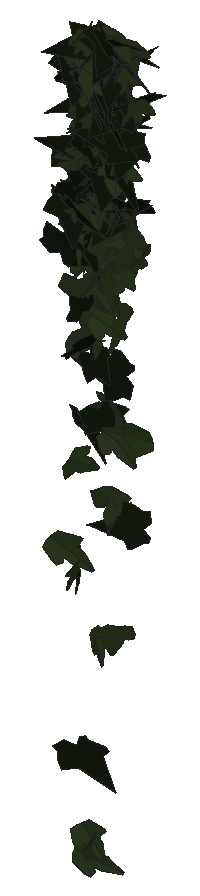
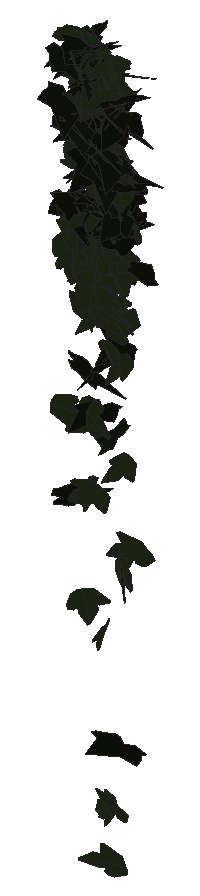
# SketchUp Ruby script. Lengths in inches.
U = 1.inch
M = Sketchup.active_model
def pt(a) = Geom::Point3d.new(a.map { |v| v * U })
def face(e, loops, mat)
  f = e.add_face(loops[0].map { |a| pt(a) })
  loops[1..].each { |l| e.add_face(l.map { |a| pt(a) }).erase! }
  f.material = f.back_material = mat if mat
  f
end
# faces: each face lists its corners as indices into pts; further lists are holes
def faces(e, pts, list, mat = nil) = list.each { |f| face(e, (f[0].is_a?(Array) ? f : [f]).map { |l| l.map { |i| pts[i] } }, mat) }
# xy, xz, yz: faces in a plane at the given z, y or x. An outline is a flat list of corners, or four numbers for a rectangle; further outlines are holes
def ring(l) = l.size == 4 ? [[l[0], l[1]], [l[2], l[1]], [l[2], l[3]], [l[0], l[3]]] : l.each_slice(2).to_a
def flat(e, list, mat, &to3) = list.each { |f| face(e, (f[0].is_a?(Array) ? f : [f]).map { |l| ring(l).map { |u, v| to3.(u, v) } }, mat) }
def xy(e, z, list, mat = nil) = flat(e, list, mat) { |x, y| [x, y, z] }
def xz(e, y, list, mat = nil) = flat(e, list, mat) { |x, z| [x, y, z] }
def yz(e, x, list, mat = nil) = flat(e, list, mat) { |y, z| [x, y, z] }
def lines(e, pts, list) = list.each { |a, b| e.add_line(pt(pts[a]), pt(pts[b])) }
# prism: a flat outline (further loops are holes) pulled along v
def prism(e, loops, v, mat = nil)
  f = face(e, loops, mat); d = Geom::Vector3d.new(v.map { |x| x * U })
  f.pushpull(f.normal.samedirection?(d) ? d.length : -d.length)
end
def box(e, o, s, mat = nil) = prism(e, [[o, [o[0] + s[0], o[1], o[2]], [o[0] + s[0], o[1] + s[1], o[2]], [o[0], o[1] + s[1], o[2]]]], [0, 0, s[2]], mat)
def at(x, y, z, deg = 0) = Geom::Transformation.translation(pt([x, y, z])) * Geom::Transformation.rotation(ORIGIN, Z_AXIS, deg.degrees)
def axes(o, x, y, z) = Geom::Transformation.new([*x, 0, *y, 0, *z, 0, *pt(o).to_a, 1])
def part(name) = M.definitions.add(name)
# library, detail: a bought-in or finely detailed component or shape, given as its bounding box
def library(name, o, s) = part(name).tap { |d| box(d.entities, o, s) }
def detail(e, o, s) = box(e.add_group.entities, o, s)
def put(e, d, t, mat = nil) = e.add_instance(d, t).tap { |i| i.material = mat if mat }
def group(e, t, mat = nil) = e.add_group.tap { |g| g.transformation = t; g.material = mat if mat }.entities
root = M.entities
M.materials.add("1026 AP 7946 SUNNY SIDE UP").color = [254, 231, 186]
M.materials.add("efeu1").color = [18, 25, 13]
M.materials.add("efeu2").color = [43, 57, 29]
c1 = part("ivyleaf_10")
p = [[0,0.5,-0.03],[-0.0625,2.02,-0.43],[-0.19,2.01,-0.46],[-0.54,1.05,-0.29],[-0.52,0.625,-0.18],[-0.83,0.76,-0.28],
  [-1.16,0.64,-0.33],[-1.15,0.33,-0.24],[-0.77,-0.39,0.02],[-0.3,-0.51,0.16],[0.04,-0.48,0.23],[-0.02,2.01,-0.4375],
  [-0.06,2.01,-0.43],[0.04,-0.49,0.23],[0.67,-0.49,0.14],[1.38,0.36,-0.2],[1.375,0.51,-0.24],[0.81,0.65,-0.19],
  [0.62,0.59,-0.15],[0.6,1.09,-0.28],[0.5,1.23,-0.31]]
faces(c1.entities,p,[[0,1,2,3,4,5,6,7,8,9,10],[11,12,0,13,14,15,16,17,18,19,20]],"efeu2")
c2 = part("ivyleaf_9")
p = [[1.54,2.16,1.25],[1.36,2.04,1.19],[-0.21,0.99,0.68],[-0.71,1.11,0.82],[-0.85,0.86,0.67],[-0.8,0.17,0.21],
  [-0.9,-0.01,0.1],[-0.67,-0.16,-0.02],[-0.08,-0.08,-0.05],[-0.03,-0.6,-0.4],[0.65,-0.88,-0.66],[0.83,-0.6,-0.49],
  [1.29,-0.42,-0.43],[1.8125,-0.07,-0.26],[1.21,0.44,0.15]]
faces(c2.entities,p,[[0,1,2,3,4,5,6,7,8,9,10,11,12,13,14]],"efeu1")
put(root,c1,axes([111.84,212.82,261.67],[0.05347,0.09968,0.2103],[-0.0247,0.20639,-0.1002],[-0.35554,0.00065,0.03859]),"1026 AP 7946 SUNNY SIDE UP")
put(root,c1,axes([111.73,212.95,262.55],[-0.1793,-0.09054,0.18329],[0.19266,0.13077,0.14979],[-0.24874,0.16655,-0.0161]),"1026 AP 7946 SUNNY SIDE UP")
put(root,c1,axes([111.68,212.8,264.51],[0.19312,-0.08424,0.20605],[0.27212,-0.10156,-0.15378],[0.20706,0.21205,0.00993]),"1026 AP 7946 SUNNY SIDE UP")
put(root,c2,axes([111.71,212.66,263.4],[-0.15918,0.06277,0.23387],[0.27221,-0.14715,0.12078],[0.25034,0.19992,0.01739]),"1026 AP 7946 SUNNY SIDE UP")
put(root,c1,axes([111.9375,212.88,265.25],[-0.22565,-0.19814,0.03871],[0.0203,-0.05639,-0.24844],[0.31679,-0.13752,0.04349]),"1026 AP 7946 SUNNY SIDE UP")
put(root,c1,axes([111.9,212.98,263.45],[0.25063,0.14947,-0.07542],[-0.0695,-0.06092,-0.22504],[-0.25292,0.16486,-0.01289]),"1026 AP 7946 SUNNY SIDE UP")
put(root,c2,axes([111.92,212.84,264.66],[0.15143,0.18297,0.13568],[0.05681,0.1277,-0.21091],[-0.34894,0.1002,0.02454]),"1026 AP 7946 SUNNY SIDE UP")
put(root,c2,axes([111.79,212.9,265.29],[-0.05234,-0.20603,-0.13394],[0.07477,0.12201,-0.21294],[0.37471,-0.05312,0.02378]),"1026 AP 7946 SUNNY SIDE UP")
put(root,c2,axes([111.87,212.83,266.68],[0.35119,0.10595,-0.05184],[-0.07077,-0.02394,-0.2548],[-0.17076,0.22783,-0.00102]),"1026 AP 7946 SUNNY SIDE UP")
put(root,c2,axes([111.77,212.91,264.72],[0.35156,-0.09277,-0.03747],[-0.06444,-0.00557,-0.2485],[0.14248,0.22637,-0.01992]),"1026 AP 7946 SUNNY SIDE UP")
put(root,c2,axes([111.86,212.72,264.35],[-0.08105,-0.23623,-0.0209],[0.00422,0.01881,-0.24897],[0.37261,-0.05159,-0.00173]),"1026 AP 7946 SUNNY SIDE UP")
put(root,c2,axes([112.11,212.61,257.58],[0.02333,-0.01712,-0.2645],[-0.35789,0.11888,-0.02103],[0.1884,0.22794,-0.0072]),"1026 AP 7946 SUNNY SIDE UP")
put(root,c2,axes([112.29,212.79,265.43],[-0.25261,0.05653,0.19369],[-0.29315,0.03089,-0.1738],[-0.0952,-0.24512,0.02123]),"1026 AP 7946 SUNNY SIDE UP")
put(root,c1,axes([112.07,212.89,263.88],[-0.3228,-0.10284,0.05543],[-0.06409,-0.03974,-0.23614],[0.17134,-0.20862,0.01609]),"1026 AP 7946 SUNNY SIDE UP")
put(root,c2,axes([112.02,212.92,265.84],[0.11278,0.23174,0.05889],[0.00151,0.05804,-0.24904],[-0.37482,0.06996,0.01672]),"1026 AP 7946 SUNNY SIDE UP")
put(root,c2,axes([111.94,212.91,266.96],[-0.17224,-0.22985,0.01436],[0.00515,-0.01844,-0.26217],[0.36217,-0.10905,0.01056]),"1026 AP 7946 SUNNY SIDE UP")
put(root,c1,axes([112.02,212.9,267.59],[0.04144,-0.25472,0.00311],[-0.00158,-0.00459,-0.26383],[0.40057,0.02633,-0.00136]),"1026 AP 7946 SUNNY SIDE UP")
put(root,c1,axes([111.7,212.58,257.88],[0.19267,0.0524,0.22442],[0.31832,0.07972,-0.13678],[-0.14992,0.23661,-0.00201]),"1026 AP 7946 SUNNY SIDE UP")
put(root,c1,axes([112.01,212.73,257.52],[0.07038,-0.22464,0.05688],[0.00922,-0.05642,-0.23624],[0.36411,0.04485,-0.00501]),"1026 AP 7946 SUNNY SIDE UP")
put(root,c1,axes([111.91,212.93,262.66],[0.29752,-0.11125,0.0746],[0.09033,-0.04626,-0.22615],[0.18878,0.19748,-0.00937]),"1026 AP 7946 SUNNY SIDE UP")
put(root,c2,axes([111.83,212.82,266.94],[0.14158,-0.2361,-0.04521],[-0.01502,0.04187,-0.26],[0.37693,0.09035,0.00662]),"1026 AP 7946 SUNNY SIDE UP")
put(root,c1,axes([112.02,212.89,263.32],[0.21001,-0.18855,0.01303],[-0.01077,-0.02161,-0.23744],[0.29707,0.13251,-0.01782]),"1026 AP 7946 SUNNY SIDE UP")
put(root,c2,axes([112.19,212.8,264.88],[-0.24343,0.18812,-0.066],[0.04972,-0.05823,-0.25102],[-0.30905,-0.15754,0.0116]),"1026 AP 7946 SUNNY SIDE UP")
put(root,c2,axes([111.75,212.65,264.375],[0.24648,-0.13163,0.16154],[0.16019,-0.12223,-0.21034],[0.28027,0.18562,-0.02184]),"1026 AP 7946 SUNNY SIDE UP")
put(root,c2,axes([112.28,212.73,266.5],[-0.33099,0.13407,-0.02675],[-0.02296,-0.07085,-0.24801],[-0.21372,-0.20001,0.06808]),"1026 AP 7946 SUNNY SIDE UP")
put(root,c1,axes([112.18,213.07,262.85],[0.0741,0.09275,-0.20945],[-0.21602,-0.15253,-0.10511],[-0.2781,0.1432,0.02584]),"1026 AP 7946 SUNNY SIDE UP")
put(root,c2,axes([112.3,212.9,267.4],[-0.34884,-0.00818,0.12883],[-0.16792,-0.12088,-0.20395],[0.10326,-0.22418,0.10357]),"1026 AP 7946 SUNNY SIDE UP")
put(root,c1,axes([112,212.62,259.56],[-0.08616,-0.13069,-0.21033],[0.16378,0.17548,-0.14401],[0.3431,-0.11658,0.01593]),"1026 AP 7946 SUNNY SIDE UP")
put(root,c1,axes([111.88,212.92,262.28],[0.18885,-0.09889,-0.17595],[0.23298,-0.08589,0.15859],[-0.20382,-0.18981,0.01826]),"1026 AP 7946 SUNNY SIDE UP")
put(root,c1,axes([112.24,212.85,261.88],[0.19717,-0.1101,-0.16509],[-0.16993,0.11815,-0.17072],[0.25317,0.16506,0.01398]),"1026 AP 7946 SUNNY SIDE UP")
put(root,c2,axes([111.98,212.89,266.46],[0.38487,-0.02762,-0.05832],[-0.08989,-0.0036,-0.25358],[0.04103,0.25116,-0.00856]),"1026 AP 7946 SUNNY SIDE UP")
put(root,c2,axes([111.92,212.83,264.56],[0.3612,-0.07913,-0.02183],[-0.01329,0.03853,-0.24767],[0.12795,0.22741,0.0359]),"1026 AP 7946 SUNNY SIDE UP")
put(root,c1,axes([112.05,212.71,264.27],[-0.2316,-0.15334,-0.12194],[0.16357,0.06154,-0.21672],[0.25595,-0.17808,0.02817]),"1026 AP 7946 SUNNY SIDE UP")
put(root,c1,axes([111.84,213.08,251.79],[0.069,0.02915,0.24774],[0.34727,0.09518,-0.05289],[-0.15585,0.22498,-0.00816]),"1026 AP 7946 SUNNY SIDE UP")
put(root,c1,axes([112.15,212.85,267.56],[0.19577,0.20167,-0.1036],[-0.1137,-0.07444,-0.24367],[-0.33646,0.1425,0.02206]),"1026 AP 7946 SUNNY SIDE UP")
put(root,c1,axes([112.22,212.73,267.1],[-0.40103,-0.03197,0.03618],[-0.04126,-0.06618,-0.25741],[0.0625,-0.24882,0.06224]),"1026 AP 7946 SUNNY SIDE UP")
put(root,c2,axes([111.89,212.8125,264.27],[0.36563,-0.00697,0.07507],[0.11244,-0.03093,-0.23816],[0.02493,0.24172,-0.02687]),"1026 AP 7946 SUNNY SIDE UP")
put(root,c1,axes([112.21,212.76,265.43],[-0.10215,-0.19356,0.14483],[-0.01668,-0.14432,-0.20898],[0.37681,-0.05886,0.03001]),"1026 AP 7946 SUNNY SIDE UP")
put(root,c1,axes([112.25,212.68,265.1875],[-0.26442,-0.16377,0.08131],[-0.06245,-0.07311,-0.24105],[0.27961,-0.1712,0.02306]),"1026 AP 7946 SUNNY SIDE UP")
put(root,c2,axes([112.37,212.9375,265.89],[-0.30157,0.15779,0.00444],[-0.02153,-0.01128,-0.25529],[-0.24723,-0.19149,0.01681]),"1026 AP 7946 SUNNY SIDE UP")
put(root,c1,axes([112.12,212.94,263.83],[-0.22432,-0.17714,-0.07376],[0.10309,0.03723,-0.2325],[0.28155,-0.15476,0.02636]),"1026 AP 7946 SUNNY SIDE UP")
put(root,c2,axes([112.33,212.42,262.63],[-0.05142,0.15685,0.1972],[-0.0844,0.18307,-0.16368],[-0.37875,-0.06209,0.0097]),"1026 AP 7946 SUNNY SIDE UP")
put(root,c2,axes([112.24,212.85,265.39],[0.07253,0.24011,0.03843],[-0.01233,0.03804,-0.2512],[-0.38155,0.04441,0.01542]),"1026 AP 7946 SUNNY SIDE UP")
put(root,c2,axes([111.96,212.93,260.19],[0.13952,-0.22077,0.07776],[0.04322,-0.07165,-0.24554],[0.36496,0.09288,-0.00065]),"1026 AP 7946 SUNNY SIDE UP")
put(root,c2,axes([111.96,212.77,254.01],[-0.06872,-0.10767,-0.23448],[0.28185,0.14808,-0.10705],[0.2768,-0.17751,0.05079]),"1026 AP 7946 SUNNY SIDE UP")
put(root,c1,axes([112.17,212.76,266.47],[-0.07146,-0.24315,-0.04562],[0.10357,0.03011,-0.24747],[0.37417,-0.05477,0.05978]),"1026 AP 7946 SUNNY SIDE UP")
put(root,c2,axes([112.05,212.82,263.71],[0.11511,-0.22771,0.03214],[-0.00401,-0.0349,-0.24625],[0.36166,0.07209,-0.01296]),"1026 AP 7946 SUNNY SIDE UP")
put(root,c2,axes([112.16,212.4375,261.83],[0.13537,0.1643,0.17037],[0.13235,0.14143,-0.19014],[-0.34071,0.12021,-0.00617]),"1026 AP 7946 SUNNY SIDE UP")
put(root,c2,axes([112.35,212.72,265.96],[-0.34043,0.09986,-0.08848],[0.10618,-0.05899,-0.24474],[-0.1785,-0.22554,0.02317]),"1026 AP 7946 SUNNY SIDE UP")
put(root,c1,axes([112.29,212.83,263.73],[-0.1663,-0.18024,0.12665],[-0.02116,-0.13207,-0.21043],[0.34332,-0.09545,0.04838]),"1026 AP 7946 SUNNY SIDE UP")
put(root,c2,axes([112.24,212.77,265.54],[-0.1233,-0.02052,0.25238],[-0.0935,-0.24804,-0.04245],[0.37527,-0.06854,0.07235]),"1026 AP 7946 SUNNY SIDE UP")
put(root,c2,axes([112.08,212.48,264.96],[0.0296,0.07848,-0.27103],[0.03559,0.26281,0.08383],[0.4309,-0.02709,0.01169]),"1026 AP 7946 SUNNY SIDE UP")
put(root,c1,axes([112.32,212.93,266.9],[-0.27535,-0.17364,0.05962],[-0.01927,-0.07012,-0.2511],[0.28765,-0.17092,0.04025]),"1026 AP 7946 SUNNY SIDE UP")
put(root,c1,axes([112.31,212.84,265.03],[-0.00973,-0.24846,-0.00336],[-0.00745,0.00197,-0.25598],[0.39062,-0.00615,-0.00497]),"1026 AP 7946 SUNNY SIDE UP")
put(root,c1,axes([112.22,212.98,263.8],[0.34949,0.06775,-0.00474],[-0.00423,-0.00826,-0.23932],[-0.10673,0.22217,-0.00603]),"1026 AP 7946 SUNNY SIDE UP")
put(root,c1,axes([112.29,212.91,266.15],[0.27581,-0.17925,0.00062],[-0.01796,-0.01344,-0.25781],[0.28129,0.1749,-0.01707]),"1026 AP 7946 SUNNY SIDE UP")
put(root,c2,axes([112.13,212.88,266.03],[0.08309,-0.2455,-0.0262],[-0.00205,0.0243,-0.25853],[0.38787,0.05272,0.00424]),"1026 AP 7946 SUNNY SIDE UP")
put(root,c2,axes([112.11,212.89,266.53],[0.06782,-0.21364,0.13321],[0.03674,-0.12843,-0.22527],[0.39194,0.049,-0.00193]),"1026 AP 7946 SUNNY SIDE UP")
put(root,c1,axes([112.37,212.8,264.4],[-0.23965,-0.1892,0.03394],[-0.01582,-0.0355,-0.25007],[0.30186,-0.15207,0.01384]),"1026 AP 7946 SUNNY SIDE UP")
put(root,c2,axes([112.32,212.84,266.76],[-0.3463,-0.11157,-0.07573],[0.15353,-0.0393,-0.24224],[0.1426,-0.22863,0.0769]),"1026 AP 7946 SUNNY SIDE UP")
put(root,c2,axes([112.625,212.85,264.625],[-0.20689,0.10198,0.18815],[-0.26569,0.07423,-0.1682],[-0.19254,-0.21201,0.02993]),"1026 AP 7946 SUNNY SIDE UP")
put(root,c1,axes([112.1875,212.82,265.93],[0.37406,-0.01364,0.07166],[0.10828,-0.0145,-0.24534],[0.02696,0.24745,-0.00897]),"1026 AP 7946 SUNNY SIDE UP")
put(root,c1,axes([112.35,212.96,264.0625],[-0.0069,-0.23705,0.01832],[-0.0017,-0.01911,-0.24436],[0.37395,-0.00446,-0.00078]),"1026 AP 7946 SUNNY SIDE UP")
put(root,c1,axes([112.39,213,263.48],[0.2437,-0.095,0.14859],[-0.17067,0.09809,0.18659],[-0.21215,-0.18804,0.02059]),"1026 AP 7946 SUNNY SIDE UP")
put(root,c1,axes([112.36,212.85,265.89],[-0.05468,-0.23538,0.08517],[0.00858,-0.08551,-0.245],[0.39288,-0.03089,0.0172]),"1026 AP 7946 SUNNY SIDE UP")
put(root,c1,axes([112.39,212.8,266.99],[-0.29771,-0.16761,0.02742],[-0.00371,-0.03869,-0.25921],[0.26707,-0.18738,0.02697]),"1026 AP 7946 SUNNY SIDE UP")
put(root,c1,axes([112.33,212.83,267.4],[0.1431,-0.23604,0.0663],[0.03641,-0.06148,-0.26097],[0.38353,0.09391,0.00003]),"1026 AP 7946 SUNNY SIDE UP")
put(root,c1,axes([112.31,212.91,263.125],[-0.03166,-0.14522,0.18632],[0.0946,-0.17941,-0.14192],[0.35328,0.03503,0.0547]),"1026 AP 7946 SUNNY SIDE UP")
put(root,c1,axes([112.32,212.8,256.22],[-0.05657,0.2325,-0.00172],[-0.01082,-0.00409,-0.24227],[-0.36545,-0.03587,0.00744]),"1026 AP 7946 SUNNY SIDE UP")
put(root,c1,axes([112.43,212.78,264.2],[-0.33045,0.10952,0.0328],[-0.09098,-0.04626,-0.23439],[-0.15424,-0.20737,0.068]),"1026 AP 7946 SUNNY SIDE UP")
put(root,c1,axes([112.45,212.77,267.51],[-0.32025,-0.14014,0.06361],[-0.04541,-0.06708,-0.25211],[0.237,-0.20222,0.03766]),"1026 AP 7946 SUNNY SIDE UP")
put(root,c2,axes([112.17,212.8,266.79],[0.06879,-0.23161,0.09249],[0.05081,-0.08643,-0.24286],[0.38803,0.05238,0.0154]),"1026 AP 7946 SUNNY SIDE UP")
put(root,c2,axes([112.26,212.76,261.58],[0.15769,-0.16483,-0.1715],[-0.08968,0.15742,-0.19616],[0.35621,0.1126,0.02654]),"1026 AP 7946 SUNNY SIDE UP")
put(root,c1,axes([112.46,212.66,262.7],[-0.41854,0.01641,-0.02349],[-0.03381,0.02209,0.27404],[0.02861,0.26625,-0.01971]),"1026 AP 7946 SUNNY SIDE UP")
put(root,c1,axes([112.45,212.86,265.26],[-0.36998,-0.07309,0.0107],[-0.00549,-0.025,-0.25288],[0.11604,-0.23421,0.02214]),"1026 AP 7946 SUNNY SIDE UP")
put(root,c2,axes([112.24,212.86,266.875],[0.08585,-0.23238,0.09558],[0.02201,-0.09333,-0.24635],[0.3936,0.05591,-0.00707]),"1026 AP 7946 SUNNY SIDE UP")
put(root,c1,axes([112.64,212.87,260.53],[0.14993,-0.05894,-0.26539],[-0.27787,0.18894,-0.11096],[0.30828,0.19897,0.02906]),"1026 AP 7946 SUNNY SIDE UP")
put(root,c1,axes([112.47,212.42,252.39],[0.05981,-0.05445,0.23149],[-0.1237,0.21143,0.06765],[-0.34237,-0.0859,0.016]),"1026 AP 7946 SUNNY SIDE UP")
put(root,c1,axes([112.49,212.61,266.28],[-0.34111,-0.13053,0.01089],[0.00137,-0.02332,-0.26011],[0.20601,-0.21598,0.01977]),"1026 AP 7946 SUNNY SIDE UP")
put(root,c2,axes([112.33,212.9,265.61],[0.30649,0.14999,0.02821],[0.05435,-0.00158,-0.25235],[-0.23326,0.19671,-0.02173]),"1026 AP 7946 SUNNY SIDE UP")
put(root,c1,axes([112.41,212.73,266.65],[0.18685,0.22195,0.00035],[-0.04362,0.01382,-0.25731],[-0.34627,0.11803,0.0326]),"1026 AP 7946 SUNNY SIDE UP")
put(root,c1,axes([112.31,212.78,264.56],[0.32717,-0.06151,0.11888],[0.15982,-0.0614,-0.2222],[0.13014,0.23004,-0.02598]),"1026 AP 7946 SUNNY SIDE UP")
put(root,c1,axes([112.52,212.91,263.79],[-0.19866,-0.19256,0.04103],[-0.01059,-0.04437,-0.23676],[0.30937,-0.12518,0.01824]),"1026 AP 7946 SUNNY SIDE UP")
put(root,c1,axes([112.23,212.62,252.59],[0.24598,0.01263,0.18063],[0.27581,-0.02524,-0.15956],[0.0165,0.23356,-0.02562]),"1026 AP 7946 SUNNY SIDE UP")
put(root,c1,axes([112.5625,212.91,262.51],[-0.43993,-0.00112,-0.01571],[-0.02404,0.01953,0.28764],[-0.00009,0.27952,-0.01852]),"1026 AP 7946 SUNNY SIDE UP")
put(root,c1,axes([112.6,212.68,263.24],[0.08561,0.18297,-0.13766],[-0.19863,-0.09071,-0.18012],[-0.29691,0.11345,0.08081]),"1026 AP 7946 SUNNY SIDE UP")
put(root,c2,axes([112.86,212.86,261.35],[-0.17483,-0.0459,-0.26275],[-0.40023,-0.03128,0.12005],[-0.07437,0.27623,-0.02839]),"1026 AP 7946 SUNNY SIDE UP")
put(root,c2,axes([112.37,212.8125,266.73],[0.06653,-0.24743,0.06433],[-0.00086,-0.06481,-0.25873],[0.40181,0.04083,-0.0112]),"1026 AP 7946 SUNNY SIDE UP")
put(root,c2,axes([112.25,212.68,266.07],[0.24403,0.01199,0.22077],[0.32944,0.04854,-0.15888],[-0.07275,0.26004,0.02106]),"1026 AP 7946 SUNNY SIDE UP")
put(root,c1,axes([112.57,212.9375,264.36],[-0.27188,-0.16671,-0.00346],[0.05805,-0.03489,-0.24206],[0.25566,-0.16937,0.05128]),"1026 AP 7946 SUNNY SIDE UP")
put(root,c1,axes([112.51,212.99,263.29],[0.09715,0.21579,0.06107],[0.0165,0.05736,-0.23084],[-0.35099,0.06243,0.00605]),"1026 AP 7946 SUNNY SIDE UP")
put(root,c1,axes([112.59,212.75,265.43],[-0.3618,0.09419,-0.01495],[0.00667,-0.02915,-0.25497],[-0.14983,-0.22874,0.02475]),"1026 AP 7946 SUNNY SIDE UP")
put(root,c1,axes([112.49,212.44,267.15],[0.05333,0.22326,0.17501],[0.03179,0.16745,-0.23163],[-0.43878,0.03927,0.00449]),"1026 AP 7946 SUNNY SIDE UP")
put(root,c2,axes([112.49,212.84,265.1],[-0.07405,-0.22935,0.0734],[0.00216,-0.07418,-0.2411],[0.37823,-0.04448,0.01574]),"1026 AP 7946 SUNNY SIDE UP")
put(root,c2,axes([112.45,212.76,260.59],[-0.00207,-0.1376,-0.21104],[0.02851,0.20347,-0.14026],[0.38596,-0.01577,0.00923]),"1026 AP 7946 SUNNY SIDE UP")
put(root,c1,axes([112.58,212.94,264.0625],[-0.34494,0.06409,-0.06517],[0.06053,-0.08482,-0.22526],[-0.12845,-0.21208,0.06884]),"1026 AP 7946 SUNNY SIDE UP")
put(root,c1,axes([112.48,212.6875,262.36],[0.07084,0.15587,0.1781],[0.09671,0.16093,-0.16589],[-0.35194,0.07559,-0.00974]),"1026 AP 7946 SUNNY SIDE UP")
put(root,c1,axes([112.46,212.89,258.9375],[-0.2714,0.00242,-0.16713],[0.2523,-0.03273,-0.17655],[-0.038,-0.23462,0.02151]),"1026 AP 7946 SUNNY SIDE UP")
put(root,c2,axes([112.71,212.9,264.43],[-0.33471,-0.11513,-0.02452],[0.05363,-0.01476,-0.24759],[0.17669,-0.21361,0.02871]),"1026 AP 7946 SUNNY SIDE UP")
put(root,c2,axes([112.59,212.88,267.19],[-0.09173,-0.24897,0.03232],[-0.00374,-0.03311,-0.26357],[0.39484,-0.05815,0.00501]),"1026 AP 7946 SUNNY SIDE UP")
put(root,c1,axes([112.72,212.72,264.42],[0.17067,-0.21377,-0.01992],[-0.03074,0.01037,-0.24658],[0.33593,0.10956,-0.01244]),"1026 AP 7946 SUNNY SIDE UP")
put(root,c2,axes([112.66,212.86,267.67],[-0.1671,-0.21306,0.09897],[-0.01853,-0.10182,-0.24361],[0.36782,-0.10192,0.03269]),"1026 AP 7946 SUNNY SIDE UP")
put(root,c2,axes([112.81,212.61,267.15],[-0.00075,0.20235,0.17131],[0.00036,0.16514,-0.20749],[-0.41069,-0.00023,-0.00049]),"1026 AP 7946 SUNNY SIDE UP")
put(root,c2,axes([112.73,212.85,266.42],[-0.26282,-0.17277,0.08773],[-0.01078,-0.10856,-0.23864],[0.30337,-0.15353,0.06752]),"1026 AP 7946 SUNNY SIDE UP")
put(root,c1,axes([112.48,212.67,263.1],[0.26604,-0.02218,0.17754],[0.26145,-0.04975,-0.17493],[0.07998,0.23642,-0.0187]),"1026 AP 7946 SUNNY SIDE UP")
put(root,c1,axes([112.73,212.96,263.47],[-0.00074,-0.23021,0.0387],[0.00973,-0.03887,-0.2373],[0.36698,0.00057,0.00637]),"1026 AP 7946 SUNNY SIDE UP")
put(root,c1,axes([112.74,212.82,267.2],[-0.40788,-0.0089,-0.00448],[0.01075,-0.08027,-0.25469],[0.01121,-0.2467,0.08143]),"1026 AP 7946 SUNNY SIDE UP")
put(root,c2,axes([112.75,212.77,267.625],[-0.22602,-0.20688,0.05216],[-0.02773,-0.05073,-0.25941],[0.3342,-0.14412,0.01375]),"1026 AP 7946 SUNNY SIDE UP")
put(root,c1,axes([112.76,212.88,264.4],[0.1521,-0.22325,0.01279],[-0.00839,-0.01721,-0.25046],[0.35159,0.09617,-0.01151]),"1026 AP 7946 SUNNY SIDE UP")
put(root,c1,axes([112.69,212.7,267.42],[0.2723,-0.18241,0.06949],[0.05979,-0.05823,-0.25916],[0.30048,0.17689,-0.0114]),"1026 AP 7946 SUNNY SIDE UP")
put(root,c2,axes([112.625,212.91,267.05],[-0.00825,-0.25046,-0.05436],[0.00648,0.05126,-0.25776],[0.40196,-0.00597,0.00304]),"1026 AP 7946 SUNNY SIDE UP")
put(root,c1,axes([112.8,212.7,267.8],[0.37706,-0.07661,-0.07471],[-0.1126,0.01256,-0.25908],[0.12116,0.25008,-0.00827]),"1026 AP 7946 SUNNY SIDE UP")
put(root,c2,axes([112.94,212.77,266.375],[-0.04618,0.2511,-0.00874],[-0.05612,-0.01404,-0.25771],[-0.39113,-0.02763,0.03801]),"1026 AP 7946 SUNNY SIDE UP")
put(root,c2,axes([112.86,212.91,264.61],[0.13977,0.19461,-0.11862],[-0.06545,-0.10873,-0.22094],[-0.35038,0.09794,-0.00605]),"1026 AP 7946 SUNNY SIDE UP")
put(root,c2,axes([112.625,212.6,267.88],[0.27557,-0.18342,-0.07633],[-0.06861,0.05928,-0.26083],[0.30276,0.18038,0.01037]),"1026 AP 7946 SUNNY SIDE UP")
put(root,c1,axes([112.71,212.8125,265.3125],[0.37816,0.05129,0.03051],[0.05207,-0.01522,-0.25243],[-0.07693,0.2418,-0.02088]),"1026 AP 7946 SUNNY SIDE UP")
put(root,c2,axes([112.63,212.84,264.6],[0.28548,-0.1626,-0.02377],[-0.04887,-0.00164,-0.25008],[0.25337,0.18289,-0.02146]),"1026 AP 7946 SUNNY SIDE UP")
put(root,c1,axes([112.88,212.67,256.59],[-0.22675,-0.18647,0.02736],[-0.00735,-0.03123,-0.24252],[0.29632,-0.14347,0.01493]),"1026 AP 7946 SUNNY SIDE UP")
put(root,c2,axes([113.17,212.6,265.93],[-0.23396,0.0789,0.19919],[-0.31687,0.00603,-0.16263],[-0.08364,-0.24355,0.05893]),"1026 AP 7946 SUNNY SIDE UP")
put(root,c2,axes([113.01,212.83,266.16],[-0.0136,0.24734,0.04553],[-0.08722,0.03987,-0.24876],[-0.38494,-0.01777,0.05476]),"1026 AP 7946 SUNNY SIDE UP")
put(root,c1,axes([112.83,212.84,263.32],[0.33651,-0.09823,-0.00186],[-0.01499,-0.01779,-0.2418],[0.15374,0.21327,-0.01951]),"1026 AP 7946 SUNNY SIDE UP")
put(root,c1,axes([113.03,212.83,264.09],[0.25298,-0.01173,-0.18033],[-0.27427,0.01396,-0.1661],[0.02865,0.23729,0.00225]),"1026 AP 7946 SUNNY SIDE UP")
put(root,c1,axes([112.89,212.88,267.43],[0.14378,-0.24213,0.00723],[-0.0051,-0.0102,-0.2666],[0.38092,0.09126,-0.0063]),"1026 AP 7946 SUNNY SIDE UP")
put(root,c1,axes([112.83,212.55,258.71],[0.02084,0.03997,-0.26493],[0.10279,0.24897,0.04475],[0.39647,-0.06665,0.00233]),"1026 AP 7946 SUNNY SIDE UP")
put(root,c1,axes([112.91,212.95,263.51],[-0.19382,-0.20041,-0.01183],[0.03814,-0.00283,-0.24133],[0.31323,-0.12366,0.02206]),"1026 AP 7946 SUNNY SIDE UP")
put(root,c2,axes([112.7,212.68,267.6875],[0.39089,0.05356,0.06214],[0.08104,0.04361,-0.25978],[-0.09711,0.25199,0.03333]),"1026 AP 7946 SUNNY SIDE UP")
put(root,c2,axes([112.74,212.84,265.32],[0.13271,-0.23551,-0.00205],[-0.00624,-0.00072,-0.25771],[0.37027,0.0844,-0.00361]),"1026 AP 7946 SUNNY SIDE UP")
put(root,c1,axes([112.95,212.89,266.58],[-0.37693,-0.07313,-0.01686],[0.03235,-0.01293,-0.25757],[0.11315,-0.2399,0.01748]),"1026 AP 7946 SUNNY SIDE UP")
put(root,c2,axes([112.81,212.63,266.22],[0.28223,-0.15519,-0.09435],[-0.1285,0.04372,-0.2434],[0.25175,0.1963,-0.01846]),"1026 AP 7946 SUNNY SIDE UP")
put(root,c1,axes([113.09,212.71,266.69],[0.08872,-0.14248,-0.22116],[-0.15213,0.19107,-0.15632],[0.37435,0.11142,-0.01111]),"1026 AP 7946 SUNNY SIDE UP")
put(root,c1,axes([113.14,212.76,264.28],[-0.25764,0.10207,0.14978],[-0.24627,0.00875,-0.18887],[-0.13022,-0.2185,0.06084]),"1026 AP 7946 SUNNY SIDE UP")
put(root,c1,axes([112.97,212.9,265.64],[-0.00602,-0.16131,0.19462],[0.01992,-0.18974,-0.16695],[0.39121,0.00718,0.0115]),"1026 AP 7946 SUNNY SIDE UP")
put(root,c1,axes([112.71,212.75,260.17],[0.25901,0.03327,0.17044],[0.2561,0.02817,-0.17292],[-0.06835,0.23162,-0.00204]),"1026 AP 7946 SUNNY SIDE UP")
put(root,c2,axes([113.14,212.79,264.53],[-0.12188,0.22308,-0.05045],[-0.02706,-0.05859,-0.241],[-0.35854,-0.07141,0.03534]),"1026 AP 7946 SUNNY SIDE UP")
put(root,c1,axes([112.99,212.62,262.42],[0.19967,-0.22146,0.00682],[-0.01025,-0.0128,-0.26277],[0.34829,0.12658,-0.01164]),"1026 AP 7946 SUNNY SIDE UP")
put(root,c1,axes([112.97,212.69,267.78],[-0.40371,-0.01071,-0.05431],[0.08383,-0.01858,-0.264],[0.01058,-0.26143,0.01945]),"1026 AP 7946 SUNNY SIDE UP")
put(root,c2,axes([112.86,212.7,267.57],[0.33926,-0.11834,-0.09176],[-0.11828,0.04665,-0.2532],[0.1999,0.22845,0.00592]),"1026 AP 7946 SUNNY SIDE UP")
put(root,c1,axes([113.11,212.69,264.21],[-0.05113,0.09701,0.25812],[-0.2034,0.21493,-0.10199],[-0.36937,-0.13178,0.02043]),"1026 AP 7946 SUNNY SIDE UP")
put(root,c2,axes([113.21,212.86,258.57],[-0.1698,-0.04331,0.22767],[-0.29617,-0.11748,-0.11909],[0.19481,-0.21635,0.0174]),"1026 AP 7946 SUNNY SIDE UP")
put(root,c2,axes([113.16,212.88,267.52],[-0.11309,0.22515,-0.10822],[0.00834,-0.10926,-0.24269],[-0.39144,-0.06738,0.02609]),"1026 AP 7946 SUNNY SIDE UP")
put(root,c1,axes([113.07,212.97,263.79],[-0.12573,-0.21652,0.04931],[-0.02009,-0.0476,-0.23801],[0.34851,-0.08085,0.00407]),"1026 AP 7946 SUNNY SIDE UP")
put(root,c2,axes([112.98,212.83,265.91],[-0.16471,-0.22565,0.02533],[-0.00016,-0.02844,-0.25617],[0.35714,-0.10408,0.01157]),"1026 AP 7946 SUNNY SIDE UP")
put(root,c1,axes([113.29,212.8,260.3125],[0.03169,0.00387,-0.24471],[-0.37341,0.00776,-0.02058],[0.01165,0.23829,0.00604]),"1026 AP 7946 SUNNY SIDE UP")
put(root,c2,axes([113.08,212.9,266.64],[0.11733,0.24049,0.00491],[-0.00359,0.00427,-0.25936],[-0.37817,0.07457,0.00399]),"1026 AP 7946 SUNNY SIDE UP")
